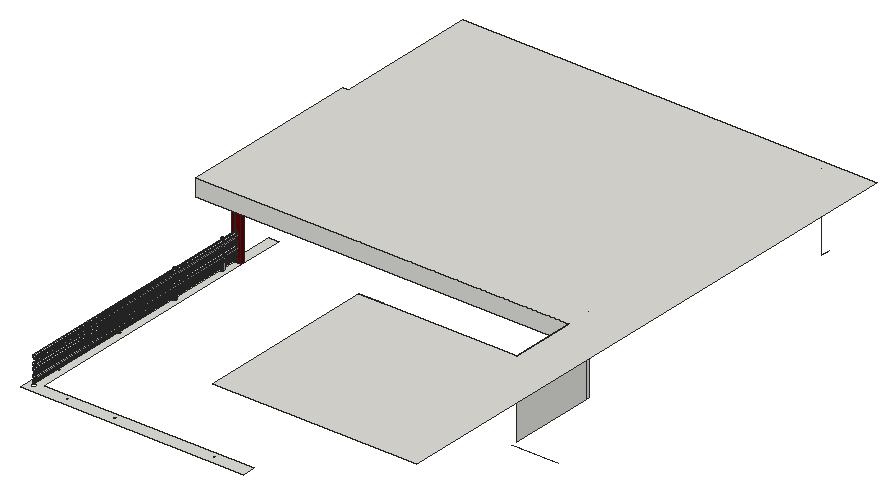
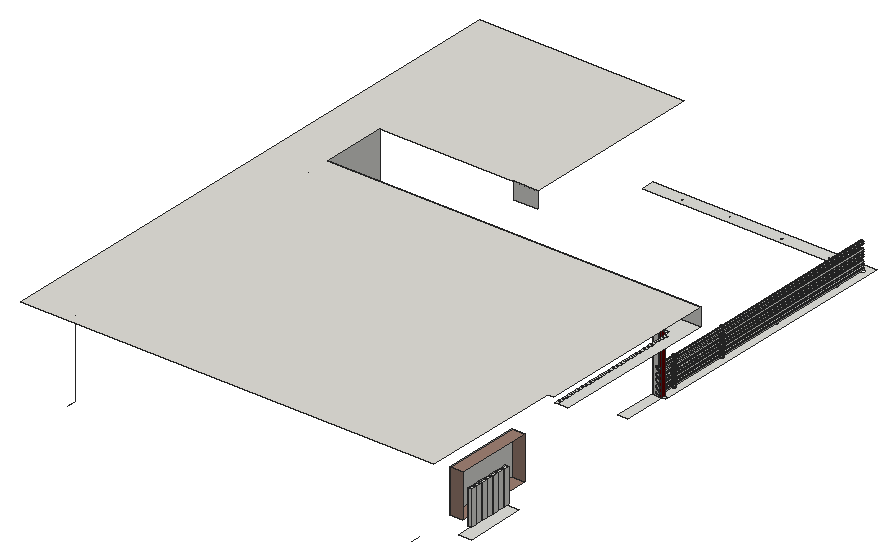
# SketchUp Ruby script. Lengths in inches.
U = 1.inch
M = Sketchup.active_model
def pt(a) = Geom::Point3d.new(a.map { |v| v * U })
def face(e, loops, mat)
  f = e.add_face(loops[0].map { |a| pt(a) })
  loops[1..].each { |l| e.add_face(l.map { |a| pt(a) }).erase! }
  f.material = f.back_material = mat if mat
  f
end
# faces: each face lists its corners as indices into pts; further lists are holes
def faces(e, pts, list, mat = nil) = list.each { |f| face(e, (f[0].is_a?(Array) ? f : [f]).map { |l| l.map { |i| pts[i] } }, mat) }
# xy, xz, yz: faces in a plane at the given z, y or x. An outline is a flat list of corners, or four numbers for a rectangle; further outlines are holes
def ring(l) = l.size == 4 ? [[l[0], l[1]], [l[2], l[1]], [l[2], l[3]], [l[0], l[3]]] : l.each_slice(2).to_a
def flat(e, list, mat, &to3) = list.each { |f| face(e, (f[0].is_a?(Array) ? f : [f]).map { |l| ring(l).map { |u, v| to3.(u, v) } }, mat) }
def xy(e, z, list, mat = nil) = flat(e, list, mat) { |x, y| [x, y, z] }
def xz(e, y, list, mat = nil) = flat(e, list, mat) { |x, z| [x, y, z] }
def yz(e, x, list, mat = nil) = flat(e, list, mat) { |y, z| [x, y, z] }
def lines(e, pts, list) = list.each { |a, b| e.add_line(pt(pts[a]), pt(pts[b])) }
# prism: a flat outline (further loops are holes) pulled along v
def prism(e, loops, v, mat = nil)
  f = face(e, loops, mat); d = Geom::Vector3d.new(v.map { |x| x * U })
  f.pushpull(f.normal.samedirection?(d) ? d.length : -d.length)
end
def box(e, o, s, mat = nil) = prism(e, [[o, [o[0] + s[0], o[1], o[2]], [o[0] + s[0], o[1] + s[1], o[2]], [o[0], o[1] + s[1], o[2]]]], [0, 0, s[2]], mat)
def at(x, y, z, deg = 0) = Geom::Transformation.translation(pt([x, y, z])) * Geom::Transformation.rotation(ORIGIN, Z_AXIS, deg.degrees)
def axes(o, x, y, z) = Geom::Transformation.new([*x, 0, *y, 0, *z, 0, *pt(o).to_a, 1])
def part(name) = M.definitions.add(name)
# library, detail: a bought-in or finely detailed component or shape, given as its bounding box
def library(name, o, s) = part(name).tap { |d| box(d.entities, o, s) }
def detail(e, o, s) = box(e.add_group.entities, o, s)
def put(e, d, t, mat = nil) = e.add_instance(d, t).tap { |i| i.material = mat if mat }
def group(e, t, mat = nil) = e.add_group.tap { |g| g.transformation = t; g.material = mat if mat }.entities
root = M.entities
M.materials.add("Niraj_Skin").color = [158, 128, 115]
M.materials.add("[Color A08]").color = [102, 0, 0]
M.materials.add("[Marble Carrara Gold Floor Tile]").color = [225, 223, 217]
xy(root,303.61,[[[86.54,109.91,294.79,109.91,294.79,121.91,98.54,121.91,98.54,355.8,98.04,355.8,98.04,352.8,92.69,352.8,92.69,355.8,89.79,355.8,89.79,352.8,86.54,352.8],[93.07,115.34,92.4375,115.35,91.82,115.52,91.28,115.84,90.83,116.29,90.51,116.84,90.35,117.46,90.36,118.1,90.53,118.71,90.85,119.26,91.3,119.7,91.85,120.02,92.47,120.18,93.11,120.18,93.72,120.01,94.27,119.69,94.72,119.23,95.03,118.68,95.19,118.0625,95.1875,117.43,95.02,116.8125,94.7,116.26,94.24,115.82,93.69,115.5],[168.99,115.46,168.62,115.51,168.27,115.65,167.97,115.88,167.74,116.18,167.6,116.52,167.55,116.89,167.6,117.27,167.74,117.61,167.97,117.91,168.27,118.14,168.62,118.28,168.99,118.33,169.36,118.28,169.71,118.14,170,117.91,170.23,117.61,170.375,117.27,170.43,116.89,170.375,116.52,170.23,116.18,170,115.88,169.71,115.65,169.36,115.51],[124.66,115.87,124.29,115.92,123.94,116.06,123.64,116.29,123.41,116.59,123.27,116.93,123.22,117.31,123.27,117.68,123.41,118.02,123.64,118.32,123.94,118.55,124.29,118.69,124.66,118.74,125.03,118.69,125.38,118.55,125.68,118.32,125.9,118.02,126.05,117.68,126.1,117.31,126.05,116.93,125.9,116.59,125.68,116.29,125.38,116.06,125.03,115.92],[261.41,115.74,261.04,115.79,260.69,115.94,260.39,116.16,260.16,116.46,260.02,116.81,259.97,117.18,260.02,117.55,260.16,117.9,260.39,118.2,260.69,118.43,261.04,118.57,261.41,118.62,261.78,118.57,262.13,118.43,262.43,118.2,262.65,117.9,262.8,117.55,262.85,117.18,262.8,116.81,262.65,116.46,262.43,116.16,262.13,115.94,261.78,115.79],[218.35,114.24,217.97,114.29,217.63,114.44,217.33,114.66,217.1,114.96,216.96,115.31,216.91,115.68,216.96,116.05,217.1,116.4,217.33,116.7,217.63,116.93,217.97,117.07,218.35,117.12,218.72,117.07,219.07,116.93,219.36,116.7,219.59,116.4,219.74,116.05,219.78,115.68,219.74,115.31,219.59,114.96,219.36,114.66,219.07,114.44,218.72,114.29],[92.88,145.7,92.51,145.75,92.16,145.89,91.87,146.12,91.64,146.42,91.49,146.76,91.44,147.14,91.49,147.51,91.64,147.86,91.87,148.15,92.16,148.38,92.51,148.53,92.88,148.57,93.25,148.53,93.6,148.38,93.9,148.15,94.13,147.86,94.27,147.51,94.32,147.14,94.27,146.76,94.13,146.42,93.9,146.12,93.6,145.89,93.25,145.75],[92.88,216.51,92.51,216.5625,92.16,216.7,91.87,216.93,91.64,217.23,91.49,217.58,91.44,217.95,91.49,218.32,91.64,218.67,91.87,218.97,92.16,219.19,92.51,219.34,92.88,219.39,93.25,219.34,93.6,219.19,93.9,218.97,94.13,218.67,94.27,218.32,94.32,217.95,94.27,217.58,94.13,217.23,93.9,216.93,93.6,216.7,93.25,216.5625],[92.88,280.39,92.51,280.4375,92.16,280.58,91.87,280.81,91.64,281.11,91.49,281.45,91.44,281.82,91.49,282.2,91.64,282.54,91.87,282.84,92.16,283.07,92.51,283.21,92.88,283.26,93.25,283.21,93.6,283.07,93.9,282.84,94.13,282.54,94.27,282.2,94.32,281.82,94.27,281.45,94.13,281.11,93.9,280.81,93.6,280.58,93.25,280.4375],[92.88,336.01,92.51,336.0625,92.16,336.2,91.87,336.43,91.64,336.73,91.49,337.08,91.44,337.45,91.49,337.82,91.64,338.17,91.87,338.47,92.16,338.69,92.51,338.84,92.88,338.89,93.25,338.84,93.6,338.69,93.9,338.47,94.13,338.17,94.27,337.82,94.32,337.45,94.27,337.08,94.13,336.73,93.9,336.43,93.6,336.2,93.25,336.0625]],[92.88,280.39,92.51,280.4375,92.16,280.58,91.87,280.81,91.64,281.11,91.49,281.45,91.44,281.82,91.49,282.2,91.64,282.54,91.87,282.84,92.16,283.07,92.51,283.21,92.88,283.26,93.25,283.21,93.6,283.07,93.9,282.84,94.13,282.54,94.27,282.2,94.32,281.82,94.27,281.45,94.13,281.11,93.9,280.81,93.6,280.58,93.25,280.4375],[86.54,352.8,89.54,355.8],[89.54,352.8,89.79,355.8],[92.69,352.8,98.04,355.8],
  [89.54,355.8,98.54,396.17]])
xy(root,304.46,[[65.54,552.74,77.54,608.18]])
xy(root,306.65,[[74.54,553.56,77.54,558.2],[74.54,559.99,77.54,564.64],[74.54,566.43,77.54,571.08],[74.54,572.87,77.54,577.51],[74.54,579.31,77.54,583.95],
  [74.54,585.74,77.54,590.39],[74.54,592.18,77.54,596.83]])
xy(root,314.17,[[77.54,530.43,89.54,603.18]],"Niraj_Skin")
xy(root,329.74,[[92.88,280.39,93.25,280.4375,93.6,280.58,93.9,280.81,94.13,281.11,94.27,281.45,94.32,281.82,94.27,282.2,94.13,282.54,93.9,282.84,93.6,283.07,93.25,283.21,92.88,283.26,92.51,283.21,92.16,283.07,91.87,282.84,91.64,282.54,91.49,282.2,91.44,281.82,91.49,281.45,91.64,281.11,91.87,280.81,92.16,280.58,92.51,280.4375]])
xy(root,330.11,[[92.88,336.01,93.25,336.0625,93.6,336.2,93.9,336.43,94.13,336.73,94.27,337.08,94.32,337.45,94.27,337.82,94.13,338.17,93.9,338.47,93.6,338.69,93.25,338.84,92.88,338.89,92.51,338.84,92.16,338.69,91.87,338.47,91.64,338.17,91.49,337.82,91.44,337.45,91.49,337.08,91.64,336.73,91.87,336.43,92.16,336.2,92.51,336.0625]])
xy(root,338.17,[[74.54,553.56,77.54,558.2],[74.54,559.99,77.54,564.64],[74.54,566.43,77.54,571.08],[74.54,572.87,77.54,577.51],[74.54,579.31,77.54,583.95],
  [74.54,585.74,77.54,590.39],[74.54,592.18,77.54,596.83]])
xy(root,354.23,[[77.54,530.43,89.54,603.18]],"Niraj_Skin")
xy(root,359.2,[[72.04,332.99,72.04,487.33,81.04,487.33,81.04,484.5625,84.04,484.5625,84.04,482.83,81.04,482.83,81.04,480.0625,84.04,480.0625,84.04,478.33,81.04,478.33,81.04,475.5625,84.04,475.5625,84.04,473.83,81.04,473.83,81.04,471.0625,84.04,471.0625,84.04,469.33,81.04,469.33,81.04,466.5625,84.04,466.5625,84.04,464.83,81.04,464.83,81.04,462.0625,84.04,462.0625,84.04,460.33,81.04,460.33,81.04,457.5625,84.04,457.5625,84.04,455.83,81.04,455.83,81.04,453.0625,84.04,453.0625,84.04,451.33,81.04,451.33,81.04,448.5625,84.04,448.5625,84.04,446.83,81.04,446.83,81.04,444.0625,84.04,444.0625,84.04,442.33,81.04,442.33,81.04,439.5625,84.04,439.5625,84.04,437.83,81.04,437.83,81.04,435.0625,84.04,435.0625,84.04,433.33,81.04,433.33,81.04,430.5625,84.04,430.5625,84.04,428.83,81.04,428.83,81.04,426.0625,84.04,426.0625,84.04,424.33,81.04,424.33,81.04,421.5625,84.04,421.5625,84.04,419.83,81.04,419.83,81.04,417.0625,84.04,417.0625,84.04,415.33,81.04,415.33,81.04,412.5625,84.04,412.5625,84.04,410.83,81.04,410.83,81.04,408.0625,84.04,408.0625,84.04,406.33,81.04,406.33,81.04,403.5625,84.04,403.5625,84.04,401.83,81.04,401.83,81.04,399.0625,84.04,399.0625,84.04,397.33,81.04,397.33,81.04,394.5625,84.04,394.5625,84.04,392.83,81.04,392.83,81.04,390.0625,84.04,390.0625,84.04,388.33,81.04,388.33,81.04,385.5625,84.04,385.5625,84.04,383.83,81.04,383.83,81.04,381.0625,84.04,381.0625,84.04,379.33,81.04,379.33,81.04,376.5625,84.04,376.5625,84.04,374.83,81.04,374.83,81.04,372.0625,84.04,372.0625,84.04,370.27,81.04,370.27,81.04,367.5,84.04,367.5,84.04,365.77,81.04,365.77,81.04,363,84.04,363,84.04,361.77,81.04,361.77,81.04,359,84.04,359,84.04,355.8,84.44,355.8,84.44,352.8,89.79,352.8,89.79,355.8,92.69,355.8,92.69,352.8,98.04,352.8,98.04,355.8,100.94,355.8,100.94,352.8,106.29,352.8,106.29,355.8,109.19,355.8,109.19,352.8,114.54,352.8,114.54,355.8,117.44,355.8,117.44,352.8,122.79,352.8,122.79,355.8,125.69,355.8,125.69,352.8,131.04,352.8,131.04,355.8,133.94,355.8,133.94,352.8,139.29,352.8,139.29,355.8,142.19,355.8,142.19,352.8,147.54,352.8,147.54,355.8,150.44,355.8,150.44,352.8,155.79,352.8,155.79,355.8,158.69,355.8,158.69,352.8,164.04,352.8,164.04,355.8,166.94,355.8,166.94,352.8,172.29,352.8,172.29,355.8,175.19,355.8,175.19,352.8,180.54,352.8,180.54,355.8,183.44,355.8,183.44,352.8,188.79,352.8,188.79,355.8,191.69,355.8,191.69,352.8,197.04,352.8,197.04,355.8,199.94,355.8,199.94,352.8,205.29,352.8,205.29,355.8,208.19,355.8,208.19,352.8,213.54,352.8,213.54,355.8,216.44,355.8,216.44,352.8,221.79,352.8,221.79,355.8,224.69,355.8,224.69,352.8,230.04,352.8,230.04,355.8,232.94,355.8,232.94,352.8,238.29,352.8,238.29,355.8,241.19,355.8,241.19,352.8,246.54,352.8,246.54,355.8,249.44,355.8,249.44,352.8,254.79,352.8,254.79,355.8,257.69,355.8,257.69,352.8,263.04,352.8,263.04,355.8,265.94,355.8,265.94,352.8,271.29,352.8,271.29,355.8,274.19,355.8,274.19,352.8,279.54,352.8,279.54,355.8,282.44,355.8,282.44,352.8,287.79,352.8,287.79,355.8,290.69,355.8,290.69,352.8,296.04,352.8,296.04,355.8,298.94,355.8,298.94,352.8,304.29,352.8,304.29,355.8,307.19,355.8,307.19,352.8,312.54,352.8,312.54,355.8,315.44,355.8,315.44,352.8,320.79,352.8,320.79,355.8,323.69,355.8,323.69,352.8,329.04,352.8,329.04,355.8,331.94,355.8,331.94,352.8,337.29,352.8,337.29,355.8,340.19,355.8,340.19,352.8,345.54,352.8,345.54,355.8,348.44,355.8,348.44,352.8,353.79,352.8,353.79,355.8,356.69,355.8,356.69,352.8,362.04,352.8,362.04,355.8,364.94,355.8,364.94,352.8,370.29,352.8,370.29,355.8,373.19,355.8,373.19,352.8,378.54,352.8,378.54,355.8,381.44,355.8,381.44,352.8,386.79,352.8,386.79,355.8,389.69,355.8,389.69,352.8,395.04,352.8,395.04,355.8,397.94,355.8,397.94,352.8,403.29,352.8,403.29,355.8,406.19,355.8,406.19,352.8,411.54,352.8,411.54,355.8,414.44,355.8,414.44,352.8,419.79,352.8,419.79,332.99],[84.44,352.8,89.54,355.8],[89.54,352.8,89.79,355.8],[92.69,352.8,98.04,355.8],[100.94,352.8,106.29,355.8],
  [109.19,352.8,114.54,355.8],[117.44,352.8,122.79,355.8],[125.69,352.8,131.04,355.8],[133.94,352.8,139.29,355.8],[142.19,352.8,147.54,355.8],
  [150.44,352.8,155.79,355.8],[158.69,352.8,164.04,355.8],[166.94,352.8,172.29,355.8],[175.19,352.8,180.54,355.8],[183.44,352.8,188.79,355.8],
  [191.69,352.8,197.04,355.8],[199.94,352.8,205.29,355.8],[208.19,352.8,213.54,355.8],[216.44,352.8,221.79,355.8],[224.69,352.8,230.04,355.8],
  [232.94,352.8,238.29,355.8],[241.19,352.8,246.54,355.8],[249.44,352.8,254.79,355.8],[257.69,352.8,263.04,355.8],[265.94,352.8,271.29,355.8],
  [274.19,352.8,279.54,355.8],[282.44,352.8,287.79,355.8],[290.69,352.8,296.04,355.8],[298.94,352.8,304.29,355.8],[307.19,352.8,312.54,355.8],
  [315.44,352.8,320.79,355.8],[323.69,352.8,329.04,355.8],[331.94,352.8,337.29,355.8],[340.19,352.8,345.54,355.8],[348.44,352.8,353.79,355.8],
  [356.69,352.8,362.04,355.8],[364.94,352.8,370.29,355.8],[373.19,352.8,378.54,355.8],[381.44,352.8,386.79,355.8],[389.69,352.8,395.04,355.8],
  [397.94,352.8,403.29,355.8],[406.19,352.8,411.54,355.8],[414.44,352.8,419.79,355.8],[81.04,359,84.04,361.77],[81.04,363,84.04,365.77],
  [81.04,367.5,84.04,370.27],[81.04,372.0625,84.04,374.83],[81.04,376.5625,84.04,379.33],[81.04,381.0625,84.04,383.83],[81.04,385.5625,84.04,388.33],
  [81.04,390.0625,84.04,392.83],[81.04,394.5625,84.04,397.33],[81.04,399.0625,84.04,401.83],[81.04,403.5625,84.04,406.33],[81.04,408.0625,83.98,410.83],
  [83.98,408.0625,84.04,410.83],[81.04,412.5625,84.04,415.33],[81.04,417.0625,84.04,419.83],[81.04,421.5625,84.04,424.33],[81.04,426.0625,84.04,428.83],
  [81.04,430.5625,84.04,433.33],[81.04,435.0625,84.04,437.83],[81.04,439.5625,84.04,442.33],[81.04,444.0625,84.04,446.83],[81.04,448.5625,84.04,451.33],
  [81.04,453.0625,84.04,455.83],[81.04,457.5625,84.04,460.33],[81.04,462.0625,84.04,464.83],[81.04,466.5625,84.04,469.33],[81.04,471.0625,84.04,473.83],
  [81.04,475.5625,84.04,478.33],[81.04,480.0625,84.04,482.83],[81.04,484.5625,84.04,487.33]])
xy(root,375.61,[[272.85,100.91,463.41,100.91,463.41,636.48,77.54,636.48,77.54,504.04,72.04,504.04,72.04,332.99,419.79,332.99,419.79,272.1,272.85,272.1]],"[Marble Carrara Gold Floor Tile]")
xz(root,272.1,[[272.85,359.87,294.79,375.61]])
xz(root,332.99,[[72.04,359.2,419.79,375.61]])
xz(root,352.8,[[92.69,303.61,98.04,303.61,98.04,359.2,92.69,359.2,92.69,329.11,92.93,329.2,93.38,329.26,93.84,329.2,94.26,329.03,94.62,328.75,94.9,328.39,95.07,327.97,95.13,327.51,95.07,327.0625,94.9,326.64,94.62,326.28,94.26,326,93.84,325.82,93.38,325.76,92.93,325.82,92.69,325.92,92.69,322.98,92.93,323.08,93.38,323.14,93.84,323.08,94.26,322.9,94.62,322.625,94.9,322.26,95.07,321.84,95.13,321.39,95.07,320.9375,94.9,320.51,94.62,320.15,94.26,319.875,93.84,319.7,93.38,319.64,92.93,319.7,92.69,319.8,92.69,318.29,92.93,318.39,93.38,318.45,93.84,318.39,94.26,318.22,94.62,317.9375,94.9,317.58,95.07,317.15,95.13,316.7,95.07,316.25,94.9,315.83,94.62,315.46,94.26,315.1875,93.84,315.01,93.38,314.95,92.93,315.01,92.69,315.11,92.69,312.79,92.93,312.89,93.38,312.95,93.84,312.89,94.26,312.72,94.62,312.4375,94.9,312.08,95.07,311.65,95.13,311.2,95.07,310.75,94.9,310.33,94.62,309.96,94.26,309.6875,93.84,309.51,93.38,309.45,92.93,309.51,92.69,309.61,92.69,307.79,92.93,307.88,93.38,307.94,93.84,307.88,94.26,307.71,94.62,307.43,94.9,307.07,95.07,306.65,95.13,306.19,95.07,305.74,94.9,305.32,94.62,304.96,94.26,304.68,93.84,304.5,93.38,304.44,92.93,304.5,92.69,304.6]],"[Color A08]")
xz(root,355.8,[[92.69,303.61,92.69,304.6,92.93,304.5,93.38,304.44,93.84,304.5,94.26,304.68,94.62,304.96,94.9,305.32,95.07,305.74,95.13,306.19,95.07,306.65,94.9,307.07,94.62,307.43,94.26,307.71,93.84,307.88,93.38,307.94,92.93,307.88,92.69,307.79,92.69,309.61,92.93,309.51,93.38,309.45,93.84,309.51,94.26,309.6875,94.62,309.96,94.9,310.33,95.07,310.75,95.13,311.2,95.07,311.65,94.9,312.08,94.62,312.4375,94.26,312.72,93.84,312.89,93.38,312.95,92.93,312.89,92.69,312.79,92.69,315.11,92.93,315.01,93.38,314.95,93.84,315.01,94.26,315.1875,94.62,315.46,94.9,315.83,95.07,316.25,95.13,316.7,95.07,317.15,94.9,317.58,94.62,317.9375,94.26,318.22,93.84,318.39,93.38,318.45,92.93,318.39,92.69,318.29,92.69,319.8,92.93,319.7,93.38,319.64,93.84,319.7,94.26,319.875,94.62,320.15,94.9,320.51,95.07,320.9375,95.13,321.39,95.07,321.84,94.9,322.26,94.62,322.625,94.26,322.9,93.84,323.08,93.38,323.14,92.93,323.08,92.69,322.98,92.69,325.92,92.93,325.82,93.38,325.76,93.84,325.82,94.26,326,94.62,326.28,94.9,326.64,95.07,327.0625,95.13,327.51,95.07,327.97,94.9,328.39,94.62,328.75,94.26,329.03,93.84,329.2,93.38,329.26,92.93,329.2,92.69,329.11,92.69,359.2,98.04,359.2,98.04,303.61],[93.38,304.44,93.84,304.5,94.26,304.68,94.62,304.96,94.9,305.32,95.07,305.74,95.13,306.19,95.07,306.65,94.9,307.07,94.62,307.43,94.26,307.71,93.84,307.88,93.38,307.94,92.93,307.88,92.69,307.79,92.69,304.6,92.93,304.5],[93.38,309.45,93.84,309.51,94.26,309.6875,94.62,309.96,94.9,310.33,95.07,310.75,95.13,311.2,95.07,311.65,94.9,312.08,94.62,312.4375,94.26,312.72,93.84,312.89,93.38,312.95,92.93,312.89,92.69,312.79,92.69,309.61,92.93,309.51],[92.69,309.61,92.69,312.79,92.51,312.72,92.15,312.4375,91.87,312.08,91.69,311.65,91.63,311.2,91.69,310.75,91.87,310.33,92.15,309.96,92.51,309.6875],[93.38,314.95,93.84,315.01,94.26,315.1875,94.62,315.46,94.9,315.83,95.07,316.25,95.13,316.7,95.07,317.15,94.9,317.58,94.62,317.9375,94.26,318.22,93.84,318.39,93.38,318.45,92.93,318.39,92.69,318.29,92.69,315.11,92.93,315.01],
  [92.69,315.11,92.69,318.29,92.51,318.22,92.15,317.9375,91.87,317.58,91.69,317.15,91.63,316.7,91.69,316.25,91.87,315.83,92.15,315.46,92.51,315.1875],[93.38,319.64,93.84,319.7,94.26,319.875,94.62,320.15,94.9,320.51,95.07,320.9375,95.13,321.39,95.07,321.84,94.9,322.26,94.62,322.625,94.26,322.9,93.84,323.08,93.38,323.14,92.93,323.08,92.69,322.98,92.69,319.8,92.93,319.7],[92.69,319.8,92.69,322.98,92.51,322.9,92.15,322.625,91.87,322.26,91.69,321.84,91.63,321.39,91.69,320.9375,91.87,320.51,92.15,320.15,92.51,319.875],[93.38,325.76,93.84,325.82,94.26,326,94.62,326.28,94.9,326.64,95.07,327.0625,95.13,327.51,95.07,327.97,94.9,328.39,94.62,328.75,94.26,329.03,93.84,329.2,93.38,329.26,92.93,329.2,92.69,329.11,92.69,325.92,92.93,325.82],[92.69,325.92,92.69,329.11,92.51,329.03,92.15,328.75,91.87,328.39,91.69,327.97,91.63,327.51,91.69,327.0625,91.87,326.64,92.15,326.28,92.51,326]])
xz(root,355.8,[[89.79,303.61,92.69,303.61,92.69,304.6,92.51,304.68,92.15,304.96,91.87,305.32,91.69,305.74,91.63,306.19,91.69,306.65,91.87,307.07,92.15,307.43,92.51,307.71,92.69,307.79,92.69,309.61,92.51,309.6875,92.15,309.96,91.87,310.33,91.69,310.75,91.63,311.2,91.69,311.65,91.87,312.08,92.15,312.4375,92.51,312.72,92.69,312.79,92.69,315.11,92.51,315.1875,92.15,315.46,91.87,315.83,91.69,316.25,91.63,316.7,91.69,317.15,91.87,317.58,92.15,317.9375,92.51,318.22,92.69,318.29,92.69,319.8,92.51,319.875,92.15,320.15,91.87,320.51,91.69,320.9375,91.63,321.39,91.69,321.84,91.87,322.26,92.15,322.625,92.51,322.9,92.69,322.98,92.69,325.92,92.51,326,92.15,326.28,91.87,326.64,91.69,327.0625,91.63,327.51,91.69,327.97,91.87,328.39,92.15,328.75,92.51,329.03,92.69,329.11,92.69,359.2,89.79,359.2]],"[Color A08]")
xz(root,530.43,[[77.54,314.17,89.54,354.23]],"Niraj_Skin")
xz(root,553.56,[[74.54,306.65,77.54,338.17]])
xz(root,558.2,[[74.54,306.65,77.54,338.17]])
xz(root,559.99,[[74.54,306.65,77.54,338.17]])
xz(root,564.64,[[74.54,306.65,77.54,338.17]])
xz(root,566.43,[[74.54,306.65,77.54,338.17]])
xz(root,571.08,[[74.54,306.65,77.54,338.17]])
xz(root,572.87,[[74.54,306.65,77.54,338.17]])
xz(root,577.51,[[74.54,306.65,77.54,338.17]])
xz(root,579.31,[[74.54,306.65,77.54,338.17]])
xz(root,583.95,[[74.54,306.65,77.54,338.17]])
xz(root,585.74,[[74.54,306.65,77.54,338.17]])
xz(root,590.39,[[74.54,306.65,77.54,338.17]])
xz(root,592.18,[[74.54,306.65,77.54,338.17]])
xz(root,596.83,[[74.54,306.65,77.54,338.17]])
xz(root,603.18,[[77.54,314.17,89.54,354.23]],"Niraj_Skin")
yz(root,74.54,[[553.56,306.65,558.2,338.17],[559.99,306.65,564.64,338.17],[566.43,306.65,571.08,338.17],[572.87,306.65,577.51,338.17],[579.31,306.65,583.95,338.17],
  [585.74,306.65,590.39,338.17],[592.18,306.65,596.83,338.17]])
yz(root,77.54,[[553.56,306.65,558.2,314.17],[559.99,306.65,564.64,314.17],[566.43,306.65,571.08,314.17],[572.87,306.65,577.51,314.17],[579.31,306.65,583.95,314.17],
  [585.74,306.65,590.39,314.17],[592.18,306.65,596.83,314.17],[553.56,314.17,558.2,338.17],[559.99,314.17,564.64,338.17],[566.43,314.17,571.08,338.17],
  [572.87,314.17,577.51,338.17],[579.31,314.17,583.95,338.17],[585.74,314.17,590.39,338.17],[592.18,314.17,596.83,338.17]])
yz(root,89.54,[[530.43,314.17,603.18,354.23]])
yz(root,89.79,[[352.8,303.61,355.8,359.2]],"[Color A08]")
yz(root,92.69,[[352.8,303.61,355.8,304.6],[352.8,307.79,355.8,309.61],[352.8,312.79,355.8,315.11],[352.8,318.29,355.8,319.8],[352.8,322.98,355.8,325.92]])
yz(root,92.69,[[352.8,329.11,355.8,359.2]],"[Color A08]")
yz(root,98.04,[[352.8,303.61,355.8,359.2]],"[Color A08]")
yz(root,419.79,[[272.1,303.61,272.1,375.61,332.99,375.61,332.99,359.2,352.8,359.2,352.8,303.61],[352.8,303.61,355.8,359.2]])
p = [[92.16,280.58,303.61],[92.51,280.4375,303.61],[92.51,280.4375,329.74],[92.16,280.58,329.74],[92.88,280.39,303.61],[92.88,280.39,329.74],
  [93.25,280.4375,303.61],[93.25,280.4375,329.74],[93.6,280.58,303.61],[93.6,280.58,329.74],[91.87,280.81,303.61],[91.87,280.81,329.74],
  [93.9,280.81,303.61],[93.9,280.81,329.74],[91.64,281.11,303.61],[91.64,281.11,329.74],[94.13,281.11,303.61],[94.13,281.11,329.74],
  [91.49,281.45,303.61],[91.49,281.45,329.74],[94.27,281.45,303.61],[94.27,281.45,329.74],[91.44,281.82,303.61],[91.44,281.82,329.74],
  [94.32,281.82,303.61],[94.32,281.82,329.74],[91.49,282.2,303.61],[91.49,282.2,329.74],[94.27,282.2,303.61],[94.27,282.2,329.74],
  [91.64,282.54,303.61],[91.64,282.54,329.74],[94.13,282.54,303.61],[94.13,282.54,329.74],[91.87,282.84,303.61],[91.87,282.84,329.74],
  [93.9,282.84,303.61],[93.9,282.84,329.74],[92.16,283.07,303.61],[92.16,283.07,329.74],[93.6,283.07,303.61],[93.6,283.07,329.74],
  [92.51,283.21,303.61],[92.51,283.21,329.74],[93.25,283.21,303.61],[93.25,283.21,329.74],[92.88,283.26,303.61],[92.88,283.26,329.74],
  [92.51,336.0625,303.61],[92.88,336.01,303.61],[92.88,336.01,330.11],[92.51,336.0625,330.11],[93.25,336.0625,303.61],[93.25,336.0625,330.11],
  [92.16,336.2,303.61],[92.16,336.2,330.11],[93.6,336.2,303.61],[93.6,336.2,330.11],[91.87,336.43,303.61],[91.87,336.43,330.11],
  [93.9,336.43,303.61],[93.9,336.43,330.11],[91.64,336.73,303.61],[91.64,336.73,330.11],[94.13,336.73,303.61],[94.13,336.73,330.11],
  [91.49,337.08,303.61],[91.49,337.08,330.11],[94.27,337.08,303.61],[94.27,337.08,330.11],[91.44,337.45,303.61],[91.44,337.45,330.11],
  [94.32,337.45,303.61],[94.32,337.45,330.11],[91.49,337.82,303.61],[91.49,337.82,330.11],[94.27,337.82,303.61],[94.27,337.82,330.11],
  [91.64,338.17,303.61],[91.64,338.17,330.11],[94.13,338.17,303.61],[94.13,338.17,330.11],[91.87,338.47,303.61],[91.87,338.47,330.11],
  [93.9,338.47,303.61],[93.9,338.47,330.11],[92.16,338.69,303.61],[92.16,338.69,330.11],[93.6,338.69,303.61],[93.6,338.69,330.11],
  [92.51,338.84,303.61],[92.51,338.84,330.11],[93.25,338.84,303.61],[93.25,338.84,330.11],[92.88,338.89,303.61],[92.88,338.89,330.11],
  [92.93,355.8,304.5],[93.38,355.8,304.44],[93.38,352.8,304.44],[92.93,352.8,304.5],[93.84,355.8,304.5],[93.84,352.8,304.5],
  [92.51,355.8,304.68],[92.69,355.8,304.6],[92.69,352.8,304.6],[92.93,118.05,304.5],[92.51,118.05,304.68],[94.26,355.8,304.68],
  [94.26,352.8,304.68],[94.62,355.8,304.96],[94.62,352.8,304.96],[94.9,355.8,305.32],[94.9,352.8,305.32],[91.69,355.8,305.74],
  [91.87,355.8,305.32],[91.87,118.05,305.32],[91.69,118.05,305.74],[95.07,355.8,305.74],[95.07,352.8,305.74],[91.63,355.8,306.19],
  [91.63,118.05,306.19],[95.13,355.8,306.19],[95.13,352.8,306.19],[91.69,355.8,306.65],[91.69,118.05,306.65],[95.07,355.8,306.65],
  [95.07,352.8,306.65],[91.87,355.8,307.07],[91.87,118.05,307.07],[94.9,355.8,307.07],[94.9,352.8,307.07],[94.62,355.8,307.43],
  [94.62,352.8,307.43],[94.26,355.8,307.71],[94.26,352.8,307.71],[92.69,355.8,307.79],[92.51,355.8,307.71],[92.51,118.05,307.71],
  [92.93,118.05,307.88],[92.93,352.8,307.88],[92.69,352.8,307.79],[93.84,355.8,307.88],[93.84,352.8,307.88],[92.93,355.8,307.88],
  [93.38,355.8,307.94],[93.38,352.8,307.94],[92.51,355.8,309.6875],[92.69,355.8,309.61],[92.69,352.8,309.61],[92.93,352.8,309.51],
  [92.93,118.05,309.51],[92.51,118.05,309.6875],[92.93,355.8,309.51],[93.38,355.8,309.45],[93.38,352.8,309.45],[93.84,355.8,309.51],
  [93.84,352.8,309.51],[94.26,355.8,309.6875],[94.26,352.8,309.6875],[92.15,355.8,309.96],[92.15,118.05,309.96],[94.62,355.8,309.96],
  [94.62,352.8,309.96],[91.87,355.8,310.33],[91.87,118.05,310.33],[94.9,355.8,310.33],[94.9,352.8,310.33],[95.07,355.8,310.75],
  [95.07,352.8,310.75],[95.07,118.05,310.75],[95.13,352.8,311.2],[95.13,118.05,311.2],[95.13,355.8,311.2],[95.07,352.8,311.65],
  [95.07,118.05,311.65],[95.07,355.8,311.65],[94.9,352.8,312.08],[94.9,118.05,312.08],[94.9,355.8,312.08],[92.15,355.8,312.4375],
  [91.87,355.8,312.08],[91.87,118.05,312.08],[92.15,118.05,312.4375],[94.62,352.8,312.4375],[94.62,118.05,312.4375],[94.62,355.8,312.4375],
  [92.51,355.8,312.72],[92.51,118.05,312.72],[94.26,352.8,312.72],[94.26,118.05,312.72],[94.26,355.8,312.72],[92.69,355.8,312.79],
  [92.93,118.05,312.89],[92.93,352.8,312.89],[92.69,352.8,312.79],[93.84,352.8,312.89],[93.84,118.05,312.89],[93.84,355.8,312.89],
  [92.93,355.8,312.89],[93.38,118.05,312.95],[93.38,352.8,312.95],[93.38,355.8,312.95],[92.51,355.8,315.1875],[92.69,355.8,315.11],
  [92.69,352.8,315.11],[92.93,352.8,315.01],[92.93,118.05,315.01],[92.51,118.05,315.1875],[93.38,352.8,314.95],[93.38,118.05,314.95],
  [93.84,352.8,315.01],[93.84,118.05,315.01],[94.26,352.8,315.1875],[94.26,118.05,315.1875],[92.93,355.8,315.01],[93.38,355.8,314.95],
  [93.84,355.8,315.01],[94.26,355.8,315.1875],[92.15,355.8,315.46],[92.15,118.05,315.46],[94.62,352.8,315.46],[94.62,118.05,315.46],
  [94.62,355.8,315.46],[91.87,355.8,315.83],[91.87,118.05,315.83],[94.9,352.8,315.83],[94.9,118.05,315.83],[94.9,355.8,315.83],
  [95.07,352.8,316.25],[95.07,118.05,316.25],[95.07,355.8,316.25],[95.13,352.8,316.7],[95.13,118.05,316.7],[95.13,355.8,316.7],
  [95.07,352.8,317.15],[95.07,118.05,317.15],[95.07,355.8,317.15],[94.9,352.8,317.58],[94.9,118.05,317.58],[94.9,355.8,317.58],
  [92.15,355.8,317.9375],[91.87,355.8,317.58],[91.87,118.05,317.58],[92.15,118.05,317.9375],[94.62,352.8,317.9375],[94.62,118.05,317.9375],
  [94.62,355.8,317.9375],[92.51,355.8,318.22],[92.51,118.05,318.22],[94.26,352.8,318.22],[94.26,118.05,318.22],[94.26,355.8,318.22],
  [92.69,355.8,318.29],[92.93,118.05,318.39],[92.93,352.8,318.39],[92.69,352.8,318.29],[93.84,352.8,318.39],[93.84,118.05,318.39],
  [93.84,355.8,318.39],[92.93,355.8,318.39],[93.38,118.05,318.45],[93.38,352.8,318.45],[93.38,355.8,318.45],[92.93,118.05,319.7],
  [92.93,352.8,319.7],[93.38,352.8,319.64],[93.38,118.05,319.64],[93.84,352.8,319.7],[93.84,118.05,319.7],[92.93,355.8,319.7],
  [93.38,355.8,319.64],[93.84,355.8,319.7],[92.51,355.8,319.875],[92.69,355.8,319.8],[92.69,352.8,319.8],[92.51,118.05,319.875],
  [94.26,352.8,319.875],[94.26,118.05,319.875],[94.26,355.8,319.875],[92.15,355.8,320.15],[92.15,118.05,320.15],[94.62,352.8,320.15],
  [94.62,118.05,320.15],[94.62,355.8,320.15],[91.87,355.8,320.51],[91.87,118.05,320.51],[94.9,352.8,320.51],[94.9,118.05,320.51],
  [94.9,355.8,320.51],[95.07,352.8,320.9375],[95.07,118.05,320.9375],[95.07,355.8,320.9375],[95.13,352.8,321.39],[95.13,118.05,321.39],
  [95.13,355.8,321.39],[95.07,352.8,321.84],[95.07,118.05,321.84],[95.07,355.8,321.84],[94.9,352.8,322.26],[94.9,118.05,322.26],
  [94.9,355.8,322.26],[92.15,355.8,322.625],[91.87,355.8,322.26],[91.87,118.05,322.26],[92.15,118.05,322.625],[94.62,352.8,322.625],
  [94.62,118.05,322.625],[94.62,355.8,322.625],[92.51,355.8,322.9],[92.51,118.05,322.9],[94.26,352.8,322.9],[94.26,118.05,322.9],
  [94.26,355.8,322.9],[92.69,355.8,322.98],[92.93,118.05,323.08],[92.93,352.8,323.08],[92.69,352.8,322.98],[93.84,352.8,323.08],
  [93.84,118.05,323.08],[93.84,355.8,323.08],[92.93,355.8,323.08],[93.38,118.05,323.14],[93.38,352.8,323.14],[93.38,355.8,323.14],
  [92.51,355.8,326],[92.69,355.8,325.92],[92.69,352.8,325.92],[92.93,352.8,325.82],[92.93,118.05,325.82],[92.51,118.05,326],
  [93.38,352.8,325.76],[93.38,118.05,325.76],[93.84,352.8,325.82],[93.84,118.05,325.82],[94.26,352.8,326],[94.26,118.05,326],
  [92.93,355.8,325.82],[93.38,355.8,325.76],[93.84,355.8,325.82],[94.26,355.8,326],[92.15,355.8,326.28],[92.15,118.05,326.28],
  [94.62,352.8,326.28],[94.62,118.05,326.28],[94.62,355.8,326.28],[91.87,355.8,326.64],[91.87,118.05,326.64],[94.9,352.8,326.64],
  [94.9,118.05,326.64],[94.9,355.8,326.64],[95.07,352.8,327.0625],[95.07,118.05,327.0625],[95.07,355.8,327.0625],[95.13,352.8,327.51],
  [95.13,118.05,327.51],[95.13,355.8,327.51],[95.07,352.8,327.97],[95.07,118.05,327.97],[95.07,355.8,327.97],[94.9,352.8,328.39],
  [94.9,118.05,328.39],[94.9,355.8,328.39],[92.15,355.8,328.75],[91.87,355.8,328.39],[91.87,118.05,328.39],[92.15,118.05,328.75],
  [94.62,352.8,328.75],[94.62,118.05,328.75],[94.62,355.8,328.75],[92.51,355.8,329.03],[92.51,118.05,329.03],[94.26,352.8,329.03],
  [94.26,118.05,329.03],[94.26,355.8,329.03],[92.69,355.8,329.11],[92.93,118.05,329.2],[92.93,352.8,329.2],[92.69,352.8,329.11],
  [93.84,352.8,329.2],[93.84,118.05,329.2],[93.84,355.8,329.2],[92.93,355.8,329.2],[93.38,118.05,329.26],[93.38,352.8,329.26],
  [93.38,355.8,329.26],[419.79,266.1,303.61],[463.41,266.1,303.61],[98.54,627.48,303.61],[98.54,636.48,303.61],[419.79,627.48,303.61],
  [419.79,636.48,303.61],[419.79,627.48,375.61],[419.79,355.8,359.2],[419.79,355.8,375.61]]
faces(root,p,[[0,1,2,3],[1,4,5,2],[4,6,7,5],[6,8,9,7],[10,0,3,11],[8,12,13,9],[14,10,11,15],[12,16,17,13],
  [18,14,15,19],[16,20,21,17],[22,18,19,23],[20,24,25,21],[26,22,23,27],[24,28,29,25],[30,26,27,31],[28,32,33,29],
  [34,30,31,35],[32,36,37,33],[38,34,35,39],[36,40,41,37],[42,38,39,43],[40,44,45,41],[46,42,43,47],[44,46,47,45],
  [48,49,50,51],[49,52,53,50],[54,48,51,55],[52,56,57,53],[58,54,55,59],[56,60,61,57],[62,58,59,63],[60,64,65,61],
  [66,62,63,67],[64,68,69,65],[70,66,67,71],[68,72,73,69],[74,70,71,75],[72,76,77,73],[78,74,75,79],[76,80,81,77],
  [82,78,79,83],[80,84,85,81],[86,82,83,87],[84,88,89,85],[90,86,87,91],[88,92,93,89],[94,90,91,95],[92,94,95,93],
  [96,97,98,99],[97,100,101,98],[102,103,104,99,105,106],[103,96,99,104],[100,107,108,101],[107,109,110,108],[109,111,112,110],[113,114,115,116],
  [111,117,118,112],[119,113,116,120],[117,121,122,118],[123,119,120,124],[121,125,126,122],[127,123,124,128],[125,129,130,126],[129,131,132,130],
  [131,133,134,132],[135,136,137,138,139,140],[133,141,142,134],[143,135,140,139],[144,143,139,145],[141,144,145,142],[146,147,148,149,150,151],[147,152,149,148],
  [152,153,154,149],[153,155,156,154],[155,157,158,156],[159,146,151,160],[157,161,162,158],[163,159,160,164],[161,165,166,162],[165,167,168,166],
  [169,168,170,171],[167,172,170,168],[171,170,173,174],[172,175,173,170],[174,173,176,177],[175,178,176,173],[179,180,181,182],[177,176,183,184],
  [178,185,183,176],[186,179,182,187],[184,183,188,189],[185,190,188,183],[191,186,187,192,193,194],[189,188,195,196],[190,197,195,188],[198,191,194,193],
  [199,200,193,192],[196,195,200,199],[201,198,193,200],[197,201,200,195],[202,203,204,205,206,207],[206,205,208,209],[209,208,210,211],[211,210,212,213],
  [203,214,205,204],[214,215,208,205],[215,216,210,208],[216,217,212,210],[218,202,207,219],[213,212,220,221],[217,222,220,212],[223,218,219,224],
  [221,220,225,226],[222,227,225,220],[226,225,228,229],[227,230,228,225],[229,228,231,232],[230,233,231,228],[232,231,234,235],[233,236,234,231],
  [235,234,237,238],[236,239,237,234],[240,241,242,243],[238,237,244,245],[239,246,244,237],[247,240,243,248],[245,244,249,250],[246,251,249,244],
  [252,247,248,253,254,255],[250,249,256,257],[251,258,256,249],[259,252,255,254],[260,261,254,253],[257,256,261,260],[262,259,254,261],[258,262,261,256],
  [263,264,265,266],[266,265,267,268],[269,270,265,264],[270,271,267,265],[272,273,274,264,263,275],[268,267,276,277],[273,269,264,274],[271,278,276,267],
  [279,272,275,280],[277,276,281,282],[278,283,281,276],[284,279,280,285],[282,281,286,287],[283,288,286,281],[287,286,289,290],[288,291,289,286],
  [290,289,292,293],[291,294,292,289],[293,292,295,296],[294,297,295,292],[296,295,298,299],[297,300,298,295],[301,302,303,304],[299,298,305,306],
  [300,307,305,298],[308,301,304,309],[306,305,310,311],[307,312,310,305],[313,308,309,314,315,316],[311,310,317,318],[312,319,317,310],[320,313,316,315],
  [321,322,315,314],[318,317,322,321],[323,320,315,322],[319,323,322,317],[324,325,326,327,328,329],[328,327,330,331],[331,330,332,333],[333,332,334,335],
  [325,336,327,326],[336,337,330,327],[337,338,332,330],[338,339,334,332],[340,324,329,341],[335,334,342,343],[339,344,342,334],[345,340,341,346],
  [343,342,347,348],[344,349,347,342],[348,347,350,351],[349,352,350,347],[351,350,353,354],[352,355,353,350],[354,353,356,357],[355,358,356,353],
  [357,356,359,360],[358,361,359,356],[362,363,364,365],[360,359,366,367],[361,368,366,359],[369,362,365,370],[367,366,371,372],[368,373,371,366],
  [374,369,370,375,376,377],[372,371,378,379],[373,380,378,371],[381,374,377,376],[382,383,376,375],[379,378,383,382],[384,381,376,383],[380,384,383,378]])
lines(root,p,[[385,386],[387,388],[389,390],[389,391],[392,393]])
